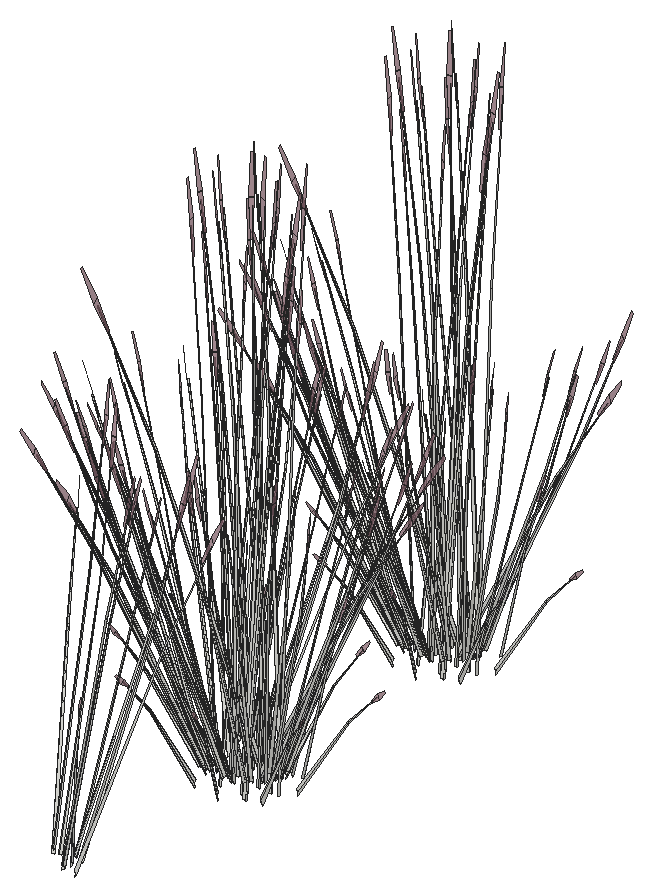
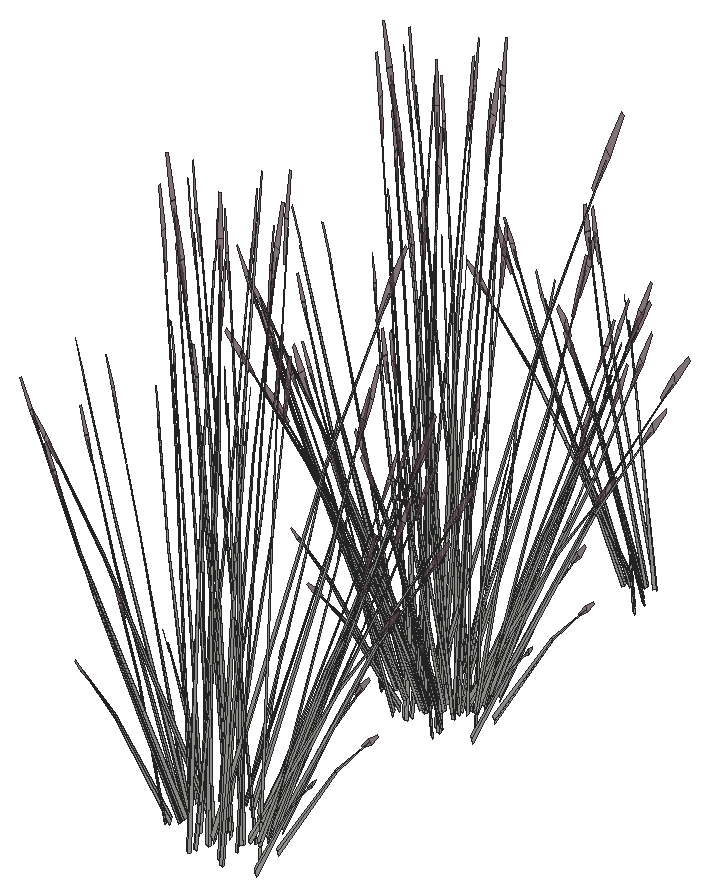
# SketchUp Ruby script. Lengths in inches.
U = 1.inch
M = Sketchup.active_model
def pt(a) = Geom::Point3d.new(a.map { |v| v * U })
def face(e, loops, mat)
  f = e.add_face(loops[0].map { |a| pt(a) })
  loops[1..].each { |l| e.add_face(l.map { |a| pt(a) }).erase! }
  f.material = f.back_material = mat if mat
  f
end
# faces: each face lists its corners as indices into pts; further lists are holes
def faces(e, pts, list, mat = nil) = list.each { |f| face(e, (f[0].is_a?(Array) ? f : [f]).map { |l| l.map { |i| pts[i] } }, mat) }
# xy, xz, yz: faces in a plane at the given z, y or x. An outline is a flat list of corners, or four numbers for a rectangle; further outlines are holes
def ring(l) = l.size == 4 ? [[l[0], l[1]], [l[2], l[1]], [l[2], l[3]], [l[0], l[3]]] : l.each_slice(2).to_a
def flat(e, list, mat, &to3) = list.each { |f| face(e, (f[0].is_a?(Array) ? f : [f]).map { |l| ring(l).map { |u, v| to3.(u, v) } }, mat) }
def xy(e, z, list, mat = nil) = flat(e, list, mat) { |x, y| [x, y, z] }
def xz(e, y, list, mat = nil) = flat(e, list, mat) { |x, z| [x, y, z] }
def yz(e, x, list, mat = nil) = flat(e, list, mat) { |y, z| [x, y, z] }
def lines(e, pts, list) = list.each { |a, b| e.add_line(pt(pts[a]), pt(pts[b])) }
# prism: a flat outline (further loops are holes) pulled along v
def prism(e, loops, v, mat = nil)
  f = face(e, loops, mat); d = Geom::Vector3d.new(v.map { |x| x * U })
  f.pushpull(f.normal.samedirection?(d) ? d.length : -d.length)
end
def box(e, o, s, mat = nil) = prism(e, [[o, [o[0] + s[0], o[1], o[2]], [o[0] + s[0], o[1] + s[1], o[2]], [o[0], o[1] + s[1], o[2]]]], [0, 0, s[2]], mat)
def at(x, y, z, deg = 0) = Geom::Transformation.translation(pt([x, y, z])) * Geom::Transformation.rotation(ORIGIN, Z_AXIS, deg.degrees)
def axes(o, x, y, z) = Geom::Transformation.new([*x, 0, *y, 0, *z, 0, *pt(o).to_a, 1])
def part(name) = M.definitions.add(name)
# library, detail: a bought-in or finely detailed component or shape, given as its bounding box
def library(name, o, s) = part(name).tap { |d| box(d.entities, o, s) }
def detail(e, o, s) = box(e.add_group.entities, o, s)
def put(e, d, t, mat = nil) = e.add_instance(d, t).tap { |i| i.material = mat if mat }
def group(e, t, mat = nil) = e.add_group.tap { |g| g.transformation = t; g.material = mat if mat }.entities
root = M.entities
M.materials.add("LightPink_Translucent").color = [144, 107, 117]
M.materials["LightPink_Translucent"].alpha = 0.75
c1 = part("blade")
p = [[2.15,0.21,22],[0,0.17,0],[0.09,0.45,0],[2.18,0.31,22],[2.29,0.31,22],[0.38,0.45,0],
  [2.48,0.24,33],[2.49,0.24,33],[2.48,0.22,33]]
faces(c1.entities,p,[[0,1,2,3],[4,5,2,3],[6,3,4,7],[8,0,3,6]])
c2 = part("seeds")
p = [[0.3,-0.1,1.38],[-0.01,-0.03,1.59],[-0.01,-0.03,0.03],[0.14,-0.07,-0.07],[0.29,-0.03,3],[0.15,0.01,3.11]]
faces(c2.entities,p,[[0,1,2,3],[1,0,4,5]],"LightPink_Translucent")
c3 = part("blade with seeds")
put(c3.entities,c1,at(0,0,0))
put(c3.entities,c2,axes([2.4,0.25,30.99],[1.5799,-0.05474,1.17369],[-0.12525,1.92788,0.29478],[-0.07173,-0.02425,1.56792]))
put(root,c3,axes([669.72,198.15,513.76],[-0.4402,0.30062,-0.29394],[-0.41671,-0.34326,0.37948],[-0.0634,0.1744,0.72609]))
put(root,c3,axes([670,199.32,512.3],[-0.01684,-0.3395,0.95334],[0.42072,0.24214,0.70045],[-0.08274,0.16182,0.20998]))
put(root,c3,axes([670.16,198.01,514.15],[0.46573,0.38364,-0.47077],[-0.49199,0.33598,-0.36465],[-0.07086,0.19492,0.90078]))
put(root,c3,axes([671.54,198.38,513.89],[0.63954,0.14313,-0.42412],[-0.21921,0.49074,-0.32852],[0.05864,0.19758,0.81151]))
put(root,c3,axes([671.9,197.37,513.22],[-0.14872,-0.18332,1.42242],[0.6872,-0.15433,0.11501],[0.15531,0.28779,0.60807]))
put(root,c3,axes([671.25,198.68,513.76],[-0.19614,0.43908,-0.29394],[-0.57222,-0.12807,0.37948],[0.05247,0.17678,0.72609]))
put(root,c3,axes([670.01,197.83,514.43],[-0.01693,0.52814,-0.65454],[-0.71285,-0.03547,0.07899],[-0.07523,0.22375,0.92591]))
put(root,c3,axes([670.6875,197.46,513.22],[-0.01592,-0.21915,1.42242],[0.69015,0.14538,0.11501],[-0.04269,0.3123,0.60807]))
put(root,c3,axes([671.3,198.28,514.13],[0.31051,0.46426,-0.58968],[-0.63919,0.25873,0.07116],[0.07261,0.22432,0.83415]))
put(root,c3,axes([669.77,198.57,512.79],[0.01429,-0.29475,1.28107],[0.64291,0.15569,0.17703],[-0.0557,0.31414,0.60492]))
put(root,c3,axes([670.27,214.07,513.22],[0.14872,0.18332,1.42242],[-0.6872,0.15433,0.11501],[-0.15531,-0.28779,0.60807]))
put(root,c3,axes([672.1,214.2,514.13],[-0.31051,-0.46426,-0.58968],[0.63919,-0.25873,0.07116],[-0.07261,-0.22432,0.83415]))
put(root,c3,axes([673.39,214.66,514.13],[0.01693,-0.52814,-0.58968],[0.71285,0.03547,0.07116],[0.07523,-0.22375,0.83415]))
put(root,c3,axes([672.16,213.81,513.76],[0.19614,-0.43908,-0.29394],[0.57222,0.12807,0.37948],[-0.05247,-0.17678,0.72609]))
put(root,c3,axes([672.59,214.39,513.22],[-0.12114,0.19625,1.42242],[-0.50818,-0.40613,0.11501],[0.22925,-0.25313,0.60807]))
put(root,c3,axes([671.87,214.11,513.89],[-0.63954,-0.14313,-0.42412],[0.21921,-0.49074,-0.32852],[-0.05864,-0.19758,0.81151]))
put(root,c3,axes([672.26,212.88,512.3],[0.08346,0.33295,0.95334],[-0.46298,-0.1844,0.70045],[0.04982,-0.17048,0.20998]))
put(root,c3,axes([673.25,214.48,513.89],[-0.46573,-0.38364,-0.42412],[0.49199,-0.33598,-0.32852],[0.07086,-0.19492,0.81151]))
put(root,c3,axes([673.69,214.34,513.76],[0.4402,-0.30062,-0.29394],[0.41671,0.34326,0.37948],[0.0634,-0.1744,0.72609]))
put(root,c3,axes([669.88,213.28,512.3],[0.33937,0.19872,0.95334],[-0.49424,0.11946,0.70045],[-0.10575,-0.15273,0.20998]))
put(root,c3,axes([670.7,214.34,514.13],[-0.55475,-0.27598,-0.58968],[0.39425,-0.48361,0.07116],[-0.20099,-0.16478,0.83415]))
put(root,c3,axes([670.51,213.97,513.76],[-0.10048,-0.4599,-0.29394],[0.5744,-0.12144,0.37948],[-0.15428,-0.13179,0.72609]))
put(root,c3,axes([669.27,214.64,513.22],[0.24166,0.09837,1.42242],[-0.50011,0.41269,0.11501],[-0.3117,-0.18617,0.60807]))
put(root,c3,axes([670.44,214.35,513.89],[-0.64198,0.13573,-0.42412],[-0.1123,-0.514,-0.32852],[-0.17243,-0.1473,0.81151]))
put(root,c3,axes([674.23,215.58,514.13],[0.33983,-0.45051,-0.58968],[0.59551,0.32017,0.07116],[0.20291,-0.16322,0.83415]))
put(root,c3,axes([674.21,215.37,513.89],[-0.16713,-0.52135,-0.42412],[0.63294,-0.0912,-0.32852],[0.18138,-0.14003,0.81151]))
put(root,c3,axes([672.03,217.46,512.76],[0.56221,0.23024,1.25546],[-0.55078,0.49601,0.49647],[-0.2467,-0.29398,1.05249]))
put(root,c3,axes([674.99,214.33,512.3],[-0.2167,0.29065,0.95334],[-0.18626,-0.3905,0.70045],[0.17898,-0.09785,0.20998]))
put(root,c3,axes([674.68,215.42,513.76],[0.56631,-0.0816,-0.29394],[0.14954,0.46647,0.37948],[0.16229,-0.12529,0.72609]))
put(root,c3,axes([669.18,214.78,513.76],[-0.37017,-0.35748,-0.29394],[0.42268,-0.3384,0.37948],[-0.21476,-0.05149,0.72609]))
put(root,c3,axes([669.57,215.02,514.13],[-0.65035,-0.01375,-0.58968],[0.04368,-0.5789,0.07116],[-0.27552,-0.06109,0.83415]))
put(root,c3,axes([669.35,215.14,513.89],[-0.47241,0.37822,-0.42412],[-0.41372,-0.39954,-0.32852],[-0.24002,-0.05755,0.81151]))
put(root,c3,axes([668.29,215.64,512.3],[0.41536,-0.04086,0.95334],[-0.26347,0.35999,0.70045],[-0.20525,-0.054,0.20998]))
put(root,c3,axes([671.22,215.97,512.26],[-0.70648,0.03525,0.37133],[-0.06389,-0.58508,-0.17871],[0.12647,-0.0593,1.19224]))
put(root,c3,axes([669.4,216.4,512.06],[0,0.57097,0.4121],[-0.72788,0,0],[0,-0.13004,1.30728]))
put(root,c3,axes([674.51,216.52,513.89],[0.17625,-0.51936,-0.42412],[0.60429,0.17802,-0.32852],[0.2433,-0.04762,0.81151]))
put(root,c3,axes([668.76,215.54,513.22],[0.26985,-0.01293,1.42242],[-0.17902,0.56047,0.11501],[-0.38456,-0.03467,0.60807]))
put(root,c3,axes([671.06,216.68,512.26],[-0.31565,0.51449,0.37133],[-0.65588,-0.24761,-0.17871],[0,-0.1186,1.19224]))
put(root,c3,axes([673.2,214.71,512.06],[-0.60889,-0.28548,0.4121],[0.36394,-0.51192,0],[0.13868,0.06502,1.30728]))
put(root,c3,axes([674.39,216.71,514.13],[0.57168,-0.25217,-0.58968],[0.3186,0.51908,0.07116],[0.27622,-0.05897,0.83415]))
put(root,c3,axes([670.89,214.97,512.05],[-0.18794,0.56744,0.14643],[-0.68774,-0.16058,0.29122],[0.1188,-0.00276,1.33138]))
put(root,c3,axes([672.07,215.73,512.26],[-0.39083,-0.47924,0.37133],[0.59199,-0.33747,-0.17871],[0.12647,0.0593,1.19224]))
put(root,c3,axes([670.83,217.89,512.05],[0.6991,-0.15154,0.14643],[0.17263,0.56398,0.29122],[-0.06235,-0.08217,1.33138]))
put(root,c3,axes([674.88,216.76,513.76],[0.54068,0.15928,-0.29394],[-0.1577,0.46469,0.37948],[0.21769,-0.04261,0.72609]))
put(root,c3,axes([668.52,216.02,513.76],[-0.54068,-0.15928,-0.29394],[0.1577,-0.46469,0.37948],[-0.21769,0.04261,0.72609]))
put(root,c3,axes([672.97,215,512.05],[-0.6991,0.15154,0.14643],[-0.17263,-0.56398,0.29122],[0.06235,0.08217,1.33138]))
put(root,c3,axes([673.41,216.1875,513.22],[-0.26985,0.01293,1.42242],[0.17902,-0.56047,0.11501],[0.38456,0.03467,0.60807]))
put(root,c3,axes([672.91,217.92,512.05],[0.18794,-0.56744,0.14643],[0.68774,0.16058,0.29122],[-0.1188,0.00276,1.33138]))
put(root,c3,axes([670.17,215.94,512.77],[0.18493,-0.0826,1.46963],[0.06377,0.5767,0.11501],[-0.40056,0.07652,0.52526]))
put(root,c3,axes([673.98,216.48,512.05],[-0.51116,-0.4159,0.14643],[0.51512,-0.4034,0.29122],[-0.05645,0.08494,1.33138]))
put(root,c3,axes([676.03,216.86,512.3],[-0.40197,0.09426,0.95334],[0.18921,-0.38956,0.70045],[0.21325,0.02666,0.20998]))
put(root,c3,axes([670.6,218.18,512.06],[0.60889,0.28548,0.4121],[-0.36394,0.51192,0],[-0.13868,-0.06502,1.30728]))
put(root,c3,axes([672.75,216.2,512.26],[0.31565,-0.51449,0.37133],[0.65588,0.24761,-0.17871],[0,0.1186,1.19224]))
put(root,c3,axes([668.89,216.26,513.89],[-0.17625,0.51936,-0.42412],[-0.60429,-0.17802,-0.32852],[-0.2433,0.04762,0.81151]))
put(root,c3,axes([675.33,218.06,513.26],[-0.12452,-0.47997,-0.02898],[0.58854,-0.11034,-0.1314],[0.1229,0.03043,0.43341]))
put(root,c3,axes([674.4,216.49,512.06],[0,-0.57097,0.4121],[0.72788,0,0],[0,0.13004,1.30728]))
put(root,c3,axes([672.58,216.92,512.26],[0.70648,-0.03525,0.37133],[0.06389,0.58508,-0.17871],[-0.12647,0.0593,1.19224]))
put(root,c3,axes([668.875,216.53,513.22],[0.22574,-0.12077,1.42242],[0.19004,0.55807,0.11501],[-0.35439,0.12613,0.60807]))
put(root,c3,axes([673.83,217.76,514.13],[0.65035,0.01375,-0.58968],[-0.04368,0.5789,0.07116],[0.27552,0.06109,0.83415]))
put(root,c3,axes([673.1,218.23,512.06],[0.60889,-0.28548,0.4121],[0.36394,0.51192,0],[-0.13868,0.06502,1.30728]))
put(root,c3,axes([667.7,218.48,512.3],[0.27113,-0.25877,0.95334],[0.10699,0.40966,0.70045],[-0.19594,0.07335,0.20998]))
put(root,c3,axes([674.23,218,513.76],[0.37017,0.35748,-0.29394],[-0.42268,0.3384,0.37948],[0.21476,0.05149,0.72609]))
put(root,c3,axes([668.72,217.36,513.76],[-0.56631,0.0816,-0.29394],[-0.14954,-0.46647,0.37948],[-0.16229,0.12529,0.72609]))
put(root,c3,axes([672.9,217.09,513.22],[-0.24166,-0.09837,1.42242],[0.50011,-0.41269,0.11501],[0.3117,0.18617,0.60807]))
put(root,c3,axes([673.79,218.21,512.3],[-0.36631,-0.16417,0.95334],[0.47299,-0.16681,0.70045],[0.12758,0.1413,0.20998]))
put(root,c3,axes([669.7,216.9,513.22],[0.1625,-0.17544,1.42242],[0.41029,0.47354,0.11501],[-0.28141,0.21565,0.60807]))
put(root,c3,axes([669.1875,217.42,513.89],[0.16713,0.52135,-0.42412],[-0.63294,0.0912,-0.32852],[-0.18138,0.14003,0.81151]))
put(root,c3,axes([672.9,216.36,512.36],[-0.01777,-0.53759,1.17256],[0.80434,0.13935,0.49647],[-0.19024,0.29416,1.1068]))
put(root,c3,axes([672.96,218.43,513.89],[0.64198,-0.13573,-0.42412],[0.1123,0.514,-0.32852],[0.17243,0.1473,0.81151]))
put(root,c3,axes([673.85,218.95,512.21],[-0.4172,-0.01791,0.872],[0.27552,-0.38032,0.48145],[0.16481,0.13512,0.68401]))
put(root,c3,axes([669.58,217.33,513.22],[0.12114,-0.19625,1.42242],[0.50818,0.40613,0.11501],[-0.22925,0.25313,0.60807]))
put(root,c3,axes([669.72,218.44,513.76],[-0.4402,0.30062,-0.29394],[-0.41671,-0.34326,0.37948],[-0.0634,0.1744,0.72609]))
put(root,c3,axes([670,219.61,512.3],[-0.01684,-0.3395,0.95334],[0.42072,0.24214,0.70045],[-0.08274,0.16182,0.20998]))
put(root,c3,axes([670.16,218.3,514.15],[0.46573,0.38364,-0.47077],[-0.49199,0.33598,-0.36465],[-0.07086,0.19492,0.90078]))
put(root,c3,axes([671.54,218.67,513.89],[0.63954,0.14313,-0.42412],[-0.21921,0.49074,-0.32852],[0.05864,0.19758,0.81151]))
put(root,c3,axes([671.9,217.66,513.22],[-0.14872,-0.18332,1.42242],[0.6872,-0.15433,0.11501],[0.15531,0.28779,0.60807]))
put(root,c3,axes([671.25,218.97,513.76],[-0.19614,0.43908,-0.29394],[-0.57222,-0.12807,0.37948],[0.05247,0.17678,0.72609]))
put(root,c3,axes([670.01,218.125,514.43],[-0.01693,0.52814,-0.65454],[-0.71285,-0.03547,0.07899],[-0.07523,0.22375,0.92591]))
put(root,c3,axes([670.6875,217.75,513.22],[-0.01592,-0.21915,1.42242],[0.69015,0.14538,0.11501],[-0.04269,0.3123,0.60807]))
put(root,c3,axes([671.3,218.58,514.13],[0.31051,0.46426,-0.58968],[-0.63919,0.25873,0.07116],[0.07261,0.22432,0.83415]))
put(root,c3,axes([669.77,218.87,512.79],[0.01429,-0.29475,1.28107],[0.64291,0.15569,0.17703],[-0.0557,0.31414,0.60492]))
put(root,c3,axes([670.27,235.77,513.22],[0.14872,0.18332,1.42242],[-0.6872,0.15433,0.11501],[-0.15531,-0.28779,0.60807]))
put(root,c3,axes([672.1,235.9,514.13],[-0.31051,-0.46426,-0.58968],[0.63919,-0.25873,0.07116],[-0.07261,-0.22432,0.83415]))
put(root,c3,axes([673.39,236.36,514.13],[0.01693,-0.52814,-0.58968],[0.71285,0.03547,0.07116],[0.07523,-0.22375,0.83415]))
put(root,c3,axes([672.16,235.51,513.76],[0.19614,-0.43908,-0.29394],[0.57222,0.12807,0.37948],[-0.05247,-0.17678,0.72609]))
put(root,c3,axes([672.59,236.09,513.22],[-0.12114,0.19625,1.42242],[-0.50818,-0.40613,0.11501],[0.22925,-0.25313,0.60807]))
put(root,c3,axes([671.87,235.81,513.89],[-0.63954,-0.14313,-0.42412],[0.21921,-0.49074,-0.32852],[-0.05864,-0.19758,0.81151]))
put(root,c3,axes([672.26,234.58,512.3],[0.08346,0.33295,0.95334],[-0.46298,-0.1844,0.70045],[0.04982,-0.17048,0.20998]))
put(root,c3,axes([673.25,236.18,513.89],[-0.46573,-0.38364,-0.42412],[0.49199,-0.33598,-0.32852],[0.07086,-0.19492,0.81151]))
put(root,c3,axes([673.69,236.04,513.76],[0.4402,-0.30062,-0.29394],[0.41671,0.34326,0.37948],[0.0634,-0.1744,0.72609]))
put(root,c3,axes([669.88,234.98,512.3],[0.33937,0.19872,0.95334],[-0.49424,0.11946,0.70045],[-0.10575,-0.15273,0.20998]))
put(root,c3,axes([670.7,236.03,514.13],[-0.55475,-0.27598,-0.58968],[0.39425,-0.48361,0.07116],[-0.20099,-0.16478,0.83415]))
put(root,c3,axes([670.51,235.67,513.76],[-0.10048,-0.4599,-0.29394],[0.5744,-0.12144,0.37948],[-0.15428,-0.13179,0.72609]))
put(root,c3,axes([669.27,236.34,513.22],[0.24166,0.09837,1.42242],[-0.50011,0.41269,0.11501],[-0.3117,-0.18617,0.60807]))
put(root,c3,axes([670.44,236.05,513.89],[-0.64198,0.13573,-0.42412],[-0.1123,-0.514,-0.32852],[-0.17243,-0.1473,0.81151]))
put(root,c3,axes([674.23,237.27,514.13],[0.33983,-0.45051,-0.58968],[0.59551,0.32017,0.07116],[0.20291,-0.16322,0.83415]))
put(root,c3,axes([674.21,237.0625,513.89],[-0.16713,-0.52135,-0.42412],[0.63294,-0.0912,-0.32852],[0.18138,-0.14003,0.81151]))
put(root,c3,axes([672.03,239.16,512.76],[0.56221,0.23024,1.25546],[-0.55078,0.49601,0.49647],[-0.2467,-0.29398,1.05249]))
put(root,c3,axes([674.99,236.03,512.3],[-0.2167,0.29065,0.95334],[-0.18626,-0.3905,0.70045],[0.17898,-0.09785,0.20998]))
put(root,c3,axes([674.68,237.12,513.76],[0.56631,-0.0816,-0.29394],[0.14954,0.46647,0.37948],[0.16229,-0.12529,0.72609]))
put(root,c3,axes([669.18,236.48,513.76],[-0.37017,-0.35748,-0.29394],[0.42268,-0.3384,0.37948],[-0.21476,-0.05149,0.72609]))
put(root,c3,axes([669.57,236.72,514.13],[-0.65035,-0.01375,-0.58968],[0.04368,-0.5789,0.07116],[-0.27552,-0.06109,0.83415]))
put(root,c3,axes([669.35,236.83,513.89],[-0.47241,0.37822,-0.42412],[-0.41372,-0.39954,-0.32852],[-0.24002,-0.05755,0.81151]))
put(root,c3,axes([668.29,237.33,512.3],[0.41536,-0.04086,0.95334],[-0.26347,0.35999,0.70045],[-0.20525,-0.054,0.20998]))
put(root,c3,axes([671.22,237.67,512.26],[-0.70648,0.03525,0.37133],[-0.06389,-0.58508,-0.17871],[0.12647,-0.0593,1.19224]))
put(root,c3,axes([669.4,238.09,512.06],[0,0.57097,0.4121],[-0.72788,0,0],[0,-0.13004,1.30728]))
put(root,c3,axes([674.51,238.22,513.89],[0.17625,-0.51936,-0.42412],[0.60429,0.17802,-0.32852],[0.2433,-0.04762,0.81151]))
put(root,c3,axes([668.76,237.24,513.22],[0.26985,-0.01293,1.42242],[-0.17902,0.56047,0.11501],[-0.38456,-0.03467,0.60807]))
put(root,c3,axes([671.06,238.38,512.26],[-0.31565,0.51449,0.37133],[-0.65588,-0.24761,-0.17871],[0,-0.1186,1.19224]))
put(root,c3,axes([673.2,236.41,512.06],[-0.60889,-0.28548,0.4121],[0.36394,-0.51192,0],[0.13868,0.06502,1.30728]))
put(root,c3,axes([674.39,238.41,514.13],[0.57168,-0.25217,-0.58968],[0.3186,0.51908,0.07116],[0.27622,-0.05897,0.83415]))
put(root,c3,axes([670.89,236.66,512.05],[-0.18794,0.56744,0.14643],[-0.68774,-0.16058,0.29122],[0.1188,-0.00276,1.33138]))
put(root,c3,axes([672.07,237.43,512.26],[-0.39083,-0.47924,0.37133],[0.59199,-0.33747,-0.17871],[0.12647,0.0593,1.19224]))
put(root,c3,axes([670.83,239.59,512.05],[0.6991,-0.15154,0.14643],[0.17263,0.56398,0.29122],[-0.06235,-0.08217,1.33138]))
put(root,c3,axes([674.88,238.46,513.76],[0.54068,0.15928,-0.29394],[-0.1577,0.46469,0.37948],[0.21769,-0.04261,0.72609]))
put(root,c3,axes([668.52,237.72,513.76],[-0.54068,-0.15928,-0.29394],[0.1577,-0.46469,0.37948],[-0.21769,0.04261,0.72609]))
put(root,c3,axes([672.97,236.69,512.05],[-0.6991,0.15154,0.14643],[-0.17263,-0.56398,0.29122],[0.06235,0.08217,1.33138]))
put(root,c3,axes([673.41,237.88,513.22],[-0.26985,0.01293,1.42242],[0.17902,-0.56047,0.11501],[0.38456,0.03467,0.60807]))
put(root,c3,axes([672.91,239.62,512.05],[0.18794,-0.56744,0.14643],[0.68774,0.16058,0.29122],[-0.1188,0.00276,1.33138]))
put(root,c3,axes([670.17,237.64,512.77],[0.18493,-0.0826,1.46963],[0.06377,0.5767,0.11501],[-0.40056,0.07652,0.52526]))
put(root,c3,axes([673.98,238.17,512.05],[-0.51116,-0.4159,0.14643],[0.51512,-0.4034,0.29122],[-0.05645,0.08494,1.33138]))
put(root,c3,axes([676.03,238.55,512.3],[-0.40197,0.09426,0.95334],[0.18921,-0.38956,0.70045],[0.21325,0.02666,0.20998]))
put(root,c3,axes([670.6,239.88,512.06],[0.60889,0.28548,0.4121],[-0.36394,0.51192,0],[-0.13868,-0.06502,1.30728]))
put(root,c3,axes([672.75,237.9,512.26],[0.31565,-0.51449,0.37133],[0.65588,0.24761,-0.17871],[0,0.1186,1.19224]))
put(root,c3,axes([668.89,237.96,513.89],[-0.17625,0.51936,-0.42412],[-0.60429,-0.17802,-0.32852],[-0.2433,0.04762,0.81151]))
put(root,c3,axes([675.33,239.75,513.26],[-0.12452,-0.47997,-0.02898],[0.58854,-0.11034,-0.1314],[0.1229,0.03043,0.43341]))
put(root,c3,axes([674.4,238.1875,512.06],[0,-0.57097,0.4121],[0.72788,0,0],[0,0.13004,1.30728]))
put(root,c3,axes([672.58,238.62,512.26],[0.70648,-0.03525,0.37133],[0.06389,0.58508,-0.17871],[-0.12647,0.0593,1.19224]))
put(root,c3,axes([668.875,238.22,513.22],[0.22574,-0.12077,1.42242],[0.19004,0.55807,0.11501],[-0.35439,0.12613,0.60807]))
put(root,c3,axes([673.83,239.46,514.13],[0.65035,0.01375,-0.58968],[-0.04368,0.5789,0.07116],[0.27552,0.06109,0.83415]))
put(root,c3,axes([673.1,239.92,512.06],[0.60889,-0.28548,0.4121],[0.36394,0.51192,0],[-0.13868,0.06502,1.30728]))
put(root,c3,axes([667.7,240.18,512.3],[0.27113,-0.25877,0.95334],[0.10699,0.40966,0.70045],[-0.19594,0.07335,0.20998]))
put(root,c3,axes([674.23,239.7,513.76],[0.37017,0.35748,-0.29394],[-0.42268,0.3384,0.37948],[0.21476,0.05149,0.72609]))
